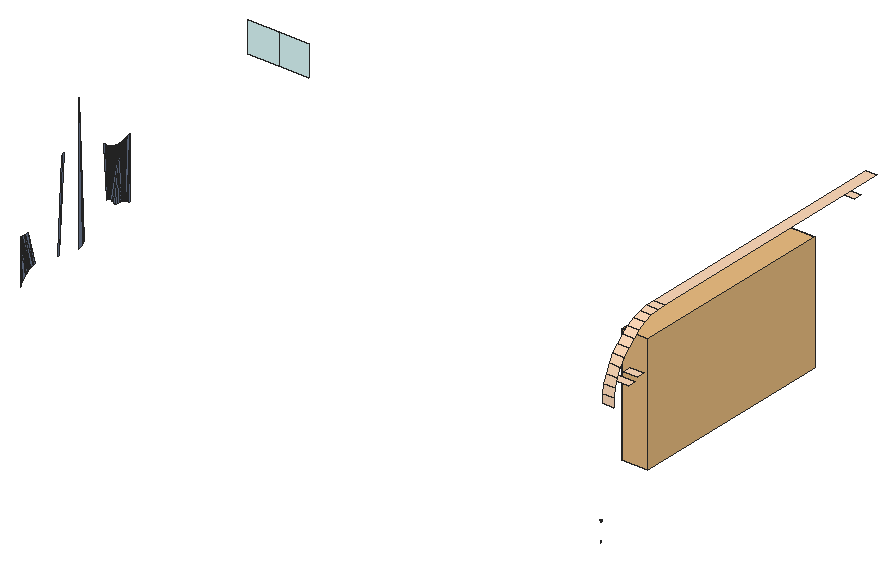
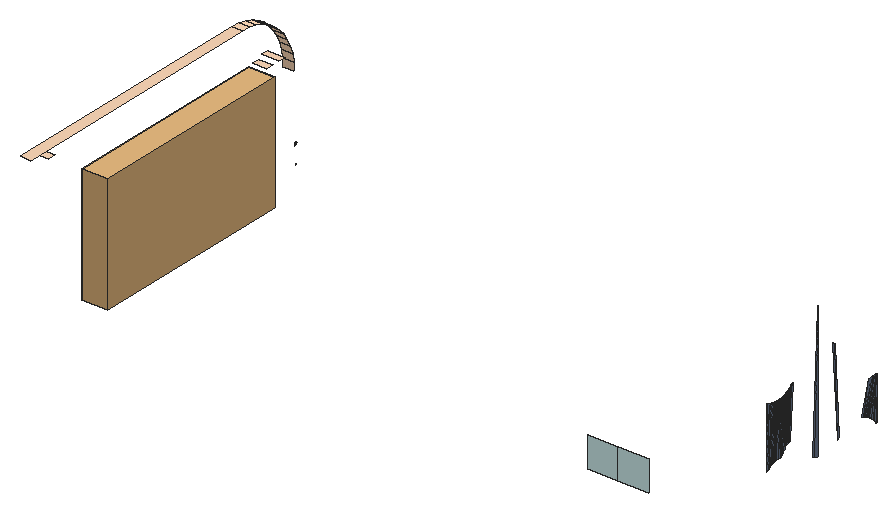
# SketchUp Ruby script. Lengths in inches.
U = 1.inch
M = Sketchup.active_model
def pt(a) = Geom::Point3d.new(a.map { |v| v * U })
def face(e, loops, mat)
  f = e.add_face(loops[0].map { |a| pt(a) })
  loops[1..].each { |l| e.add_face(l.map { |a| pt(a) }).erase! }
  f.material = f.back_material = mat if mat
  f
end
# faces: each face lists its corners as indices into pts; further lists are holes
def faces(e, pts, list, mat = nil) = list.each { |f| face(e, (f[0].is_a?(Array) ? f : [f]).map { |l| l.map { |i| pts[i] } }, mat) }
# xy, xz, yz: faces in a plane at the given z, y or x. An outline is a flat list of corners, or four numbers for a rectangle; further outlines are holes
def ring(l) = l.size == 4 ? [[l[0], l[1]], [l[2], l[1]], [l[2], l[3]], [l[0], l[3]]] : l.each_slice(2).to_a
def flat(e, list, mat, &to3) = list.each { |f| face(e, (f[0].is_a?(Array) ? f : [f]).map { |l| ring(l).map { |u, v| to3.(u, v) } }, mat) }
def xy(e, z, list, mat = nil) = flat(e, list, mat) { |x, y| [x, y, z] }
def xz(e, y, list, mat = nil) = flat(e, list, mat) { |x, z| [x, y, z] }
def yz(e, x, list, mat = nil) = flat(e, list, mat) { |y, z| [x, y, z] }
def lines(e, pts, list) = list.each { |a, b| e.add_line(pt(pts[a]), pt(pts[b])) }
# prism: a flat outline (further loops are holes) pulled along v
def prism(e, loops, v, mat = nil)
  f = face(e, loops, mat); d = Geom::Vector3d.new(v.map { |x| x * U })
  f.pushpull(f.normal.samedirection?(d) ? d.length : -d.length)
end
def box(e, o, s, mat = nil) = prism(e, [[o, [o[0] + s[0], o[1], o[2]], [o[0] + s[0], o[1] + s[1], o[2]], [o[0], o[1] + s[1], o[2]]]], [0, 0, s[2]], mat)
def at(x, y, z, deg = 0) = Geom::Transformation.translation(pt([x, y, z])) * Geom::Transformation.rotation(ORIGIN, Z_AXIS, deg.degrees)
def axes(o, x, y, z) = Geom::Transformation.new([*x, 0, *y, 0, *z, 0, *pt(o).to_a, 1])
def part(name) = M.definitions.add(name)
# library, detail: a bought-in or finely detailed component or shape, given as its bounding box
def library(name, o, s) = part(name).tap { |d| box(d.entities, o, s) }
def detail(e, o, s) = box(e.add_group.entities, o, s)
def put(e, d, t, mat = nil) = e.add_instance(d, t).tap { |i| i.material = mat if mat }
def group(e, t, mat = nil) = e.add_group.tap { |g| g.transformation = t; g.material = mat if mat }.entities
root = M.entities
M.materials.add("3D66_SU_1584934530605_002").color = [112, 126, 151]
M.materials.add("Material \#1").color = [140, 140, 140]
M.materials.add("[0027_PeachPuff]").color = [255, 218, 185]
M.materials.add("[0090_LightCyan]").color = [224, 255, 255]
c1 = library("Flat screen television",[0,1.41,1.14],[35.92,0.28,20.21])
xy(root,94.84,[[354.3125,217.7,361.25,220.7],[354.3125,223.77,359.875,226.77]],"[0027_PeachPuff]")
xy(root,110.27,[[354.3125,330.97,359.375,333.97]],"[0027_PeachPuff]")
xy(root,113.35,[[354.3125,238.49,358.5625,342.58]],"[0027_PeachPuff]")
xz(root,333.9375,[[118.5625,75.41,130.5625,87.41],[130.5625,75.41,142.5625,87.41]],"[0090_LightCyan]")
yz(root,123.07,[[216.34,46.75,216.58,47.05,216.82,47.36],[216.34,46.75,216.82,47.36,216.34,64.1875],[216.82,47.36,217.29,47.98,216.34,64.1875],[216.82,47.36,217.06,47.67,217.29,47.98],[244.87,47.51,246.34,48.07,244.87,100.53],
  [217.29,47.98,217.81,48.58,216.34,64.1875],[217.29,47.98,217.54,48.28,217.81,48.58],[246.34,48.07,247.03,48.37,244.87,100.53],[247.03,48.37,247.68,48.68,244.87,100.53],[217.81,48.58,218.42,49.17,216.34,64.1875],
  [217.81,48.58,218.1,48.875,218.42,49.17],[218.42,49.17,219.12,49.77,216.34,64.1875],[218.42,49.17,218.76,49.47,219.12,49.77],[235.3125,49.2,236.83,83.75,234.68,49.63],[235.3125,49.2,237.76,84.43,236.83,83.75],
  [219.12,49.77,219.86,50.33,216.34,64.1875],[219.12,49.77,219.49,50.06,219.86,50.33],[219.86,50.33,220.23,50.58,216.34,64.1875],[220.23,50.58,216.63,64.11,216.34,64.1875],[220.23,50.58,220.59,50.81,216.63,64.11],
  [220.59,50.81,216.92,64.05,216.63,64.11],[220.59,50.81,220.9375,51.01,216.92,64.05],[220.9375,51.01,217.23,63.99,216.92,64.05],[220.9375,51.01,217.84,63.92,217.23,63.99],[220.9375,51.01,218.15,63.9,217.84,63.92],
  [220.9375,51.01,221.3,51.18,218.15,63.9],[221.3,51.18,218.47,63.89,218.15,63.9],[221.3,51.18,221.65,51.34,218.47,63.89],[221.65,51.34,222.35,51.6,218.47,63.89],[221.65,51.34,222,51.48,222.35,51.6],
  [222.35,51.6,222.6875,51.7,218.47,63.89],[222.6875,51.7,220.09,64.05,218.47,63.89],[222.6875,51.7,223.3125,51.87,220.09,64.05],[222.6875,51.7,223.01,51.79,223.3125,51.87],[269.95,53.02,269.95,77.01,269.54,53.4],
  [269.54,53.4,269.95,77.01,269.33,53.58],[269.33,53.58,269.95,77.01,269.11,53.75],[269.11,53.75,269.95,77.01,268.89,53.9],[268.89,53.9,269.95,77.01,268.66,54.05],[268.19,54.33,269.95,77.01,268.79,76.57],
  [267.48,54.67,268.79,76.57,268.2,76.37],[267.23,54.76,268.2,76.37,267.6,76.18],[266.71,54.93,267.6,76.18,266.99,76.03],[266.43,55,266.68,75.97,266.13,55.07],[266.43,55,266.99,76.03,266.68,75.97],
  [266.13,55.07,266.37,75.91,266.05,55.09],[266.13,55.07,266.68,75.97,266.37,75.91],[266.05,55.09,266.37,75.91,265.97,55.1],[265.97,55.1,266.05,75.87,265.79,55.12],[265.97,55.1,266.37,75.91,266.05,75.87],
  [265.79,55.12,265.72,75.84,265.61,55.13],[265.79,55.12,266.05,75.87,265.72,75.84],[265.61,55.13,265.4,75.82,265.43,55.14],[265.61,55.13,265.72,75.84,265.4,75.82],[265.43,55.14,265.06,75.81,264.64,55.15],
  [265.43,55.14,265.4,75.82,265.06,75.81],[264.64,55.15,265.06,75.81,264.24,55.16],[264.24,55.16,265.06,75.81,264.05,55.18],[264.05,55.18,265.06,75.81,263.86,55.2],[263.86,55.2,265.06,75.81,263.76,55.22],
  [263.76,55.22,265.06,75.81,263.67,55.24],[263.67,55.24,265.06,75.81,263.58,55.26],[263.58,55.26,265.06,75.81,263.49,55.28],[263.49,55.28,265.06,75.81,263.41,55.31],[263.41,55.31,265.06,75.81,263.32,55.34],
  [263.32,55.34,265.06,75.81,263.24,55.37],[263.24,55.37,265.06,75.81,263.16,55.41],[263.16,55.41,265.06,75.81,263.09,55.45],[263.09,55.45,265.06,75.81,263.01,55.5],[263.01,55.5,265.06,75.81,262.94,55.55],
  [262.94,55.55,265.06,75.81,262.87,55.61],[262.87,55.61,265.06,75.81,262.8,55.66],[262.8,55.66,265.06,75.81,262.73,55.73],[262.73,55.73,265.06,75.81,262.6,55.86],[262.6,55.86,265.06,75.81,262.47,56],
  [262.47,56,265.06,75.81,262.35,56.15],[262.35,56.15,265.06,75.81,262.11,56.47],[262.11,56.47,265.06,75.81,261.65,57.11],[261.65,57.11,265.06,75.81,261.53,57.26],[261.53,57.26,265.06,75.81,261.41,57.4],
  [261.41,57.4,265.06,75.81,261.29,57.52],[261.29,57.52,265.06,75.81,261.23,57.58],[261.23,57.58,265.06,75.81,261.17,57.64],[261.17,57.64,265.06,75.81,260.66,58.06],[260.66,58.06,265.06,75.81,260.4,58.25],
  [260.4,58.25,265.06,75.81,260.14,58.42],[260.14,58.42,265.06,75.81,259.88,58.58],[259.88,58.58,265.06,75.81,259.76,58.65],[259.76,58.65,265.06,75.81,259.63,58.71],[259.63,58.71,264.58,75.82,259.5,58.77],
  [259.63,58.71,265.06,75.81,264.58,75.82],[259.5,58.77,264.58,75.82,259.375,58.8125],[259.375,58.8125,264.1,75.85,259.25,58.85],[259.375,58.8125,264.58,75.82,264.1,75.85],[259.25,58.85,263.63,75.9,259.1875,58.87],
  [259.25,58.85,264.1,75.85,263.63,75.9],[259.1875,58.87,263.63,75.9,259.125,58.89],[259.125,58.89,263.17,75.97,259.07,58.9],[259.125,58.89,263.63,75.9,263.17,75.97],[259.07,58.9,263.17,75.97,259,58.91],
  [259,58.91,262.72,76.05,258.94,58.92],[259,58.91,263.17,75.97,262.72,76.05],[258.625,58.92,257.83,78.65,257.55,78.95],[258.625,58.92,258.12,78.37,257.83,78.65],[258.625,58.92,258.43,78.1,258.12,78.37],
  [258.625,58.92,258.76,77.84,258.43,78.1],[258.625,58.92,258.6875,58.93,261.84,76.28],[258.625,58.92,259.1,77.59,258.76,77.84],[258.625,58.92,259.45,77.36,259.1,77.59],[258.625,58.92,259.82,77.14,259.45,77.36],
  [258.625,58.92,260.2,76.94,259.82,77.14],[258.625,58.92,260.59,76.75,260.2,76.94],[258.625,58.92,261,76.58,260.59,76.75],[258.625,58.92,261.41,76.42,261,76.58],[258.625,58.92,261.84,76.28,261.41,76.42],
  [258.88,58.92,262.27,76.16,258.8125,58.93],[258.88,58.92,258.94,58.92,262.72,76.05],[258.88,58.92,262.72,76.05,262.27,76.16],[258.6875,58.93,258.75,58.93,261.84,76.28],[258.75,58.93,258.8125,58.93,262.27,76.16],
  [258.75,58.93,262.27,76.16,261.84,76.28],[217.84,63.92,217.53,63.95,217.23,63.99]],"3D66_SU_1584934530605_002")
yz(root,362.5625,[[201.98,47.07,201.99,47.07,202.1,47.3],[201.99,47.07,202.04,47.14,202.1,47.3],[202.04,47.14,202.07,47.17,202.08,47.21],[202.04,47.14,202.08,47.21,202.1,47.3],[202.01,47.15,202.1,47.3,202.04,47.21],
  [202.04,47.21,202.1,47.3,202.0625,47.27],[202.08,47.21,202.09,47.25,202.1,47.3],[202.0625,47.27,202.1,47.3,202.07,47.34],[202.1,47.3,202.04,47.55,202.0625,47.41],[202.1,47.3,202.1,47.42,202.04,47.55],
  [202.1,47.3,202.0625,47.41,202.07,47.34],[202.1,47.3,202.11,47.34,202.1,47.42]],"Material \#1")
yz(root,362.57,[[202.58,54.24,202.58,54.4,202.5625,54.4],[202.58,54.24,202.59,54.24,202.58,54.4],[202.5625,54.4,202.54,54.54,202.53,54.54],[202.5625,54.4,202.58,54.4,202.54,54.54],[202.02,54.44,202.04,54.49,202.01,54.45],
  [202.01,54.45,202.04,54.49,202.03,54.49],[202.03,54.49,202.04,54.49,202.06,54.54],[202.03,54.49,202.06,54.54,202.04,54.54],[202.04,54.54,202.06,54.54,202.0625,54.6],[202.04,54.54,202.0625,54.6,202.05,54.6],
  [202.53,54.54,202.48,54.68,202.47,54.67],[202.53,54.54,202.54,54.54,202.48,54.68],[202.05,54.6,202.06,54.64,202.04,54.64],[202.05,54.6,202.0625,54.6,202.06,54.64],[202.04,54.64,202.04,54.6875,202.03,54.68],
  [202.04,54.64,202.06,54.64,202.04,54.6875],[202.47,54.67,202.4,54.8,202.39,54.79],[202.47,54.67,202.48,54.68,202.4,54.8],[202.03,54.68,202.02,54.73,202.01,54.73],[202.03,54.68,202.04,54.6875,202.02,54.73],
  [202.39,54.79,202.31,54.9,202.3,54.89],[202.39,54.79,202.4,54.8,202.31,54.9],[202.3,54.89,202.2,54.99,202.19,54.98],[202.3,54.89,202.31,54.9,202.2,54.99],[202.19,54.98,202.07,55.05,202.07,55.04],
  [202.19,54.98,202.2,54.99,202.07,55.05],[202.07,55.04,202.07,55.05,201.94,55.09]],"Material \#1")
yz(root,362.58,[[201.98,47.0625,202.01,47.15,202.04,47.21],[201.98,47.0625,202.04,47.21,202.1,47.3],[201.98,47.0625,202.1,47.3,201.98,47.07],[201.98,47.07,202.1,47.3,201.99,47.07],[201.99,47.07,202.04,47.14,201.99,47.08],
  [201.99,47.07,202.1,47.3,202.04,47.14],[201.99,47.08,202.04,47.14,202.02,47.11],[202.04,47.14,202.08,47.21,202.07,47.17],[202.04,47.14,202.1,47.3,202.08,47.21],[202.04,47.21,202.0625,47.27,202.1,47.3],
  [202.08,47.21,202.1,47.3,202.09,47.25],[202.0625,47.27,202.07,47.34,202.1,47.3],[202.1,47.3,202.04,47.47,202.04,47.55],[202.1,47.3,202.04,47.55,202.1,47.42],[202.1,47.3,202.0625,47.41,202.04,47.47],
  [202.1,47.3,202.07,47.34,202.0625,47.41],[202.1,47.3,202.1,47.42,202.11,47.34],[202.1,47.42,202.04,47.55,202.07,47.49]],"Material \#1")
yz(root,362.67,[[201.98,47.0625,202.1,47.3,202.04,47.21],[201.98,47.07,201.99,47.07,202.1,47.3],[201.99,47.07,202.04,47.14,202.1,47.3],[202.04,47.14,202.07,47.17,202.08,47.21],[202.04,47.14,202.08,47.21,202.1,47.3],
  [202.04,47.21,202.1,47.3,202.0625,47.27],[202.08,47.21,202.09,47.25,202.1,47.3],[202.0625,47.27,202.1,47.3,202.07,47.34],[202.1,47.3,202.04,47.47,202.0625,47.41],[202.1,47.3,202.04,47.55,202.04,47.47],
  [202.1,47.3,202.1,47.42,202.04,47.55],[202.1,47.3,202.0625,47.41,202.07,47.34],[202.1,47.3,202.11,47.34,202.1,47.42],[202.1,47.42,202.07,47.49,202.04,47.55],[202.04,47.47,202.04,47.55,202.01,47.52]],"Material \#1")
yz(root,362.6875,[[201.98,47.07,202.1,47.3,201.99,47.07],[201.99,47.07,202.1,47.3,202.04,47.14],[202.04,47.14,202.08,47.21,202.07,47.17],[202.04,47.14,202.1,47.3,202.08,47.21],[202.01,47.15,202.04,47.21,202.1,47.3],
  [202.04,47.21,202.0625,47.27,202.1,47.3],[202.08,47.21,202.1,47.3,202.09,47.25],[202.0625,47.27,202.07,47.34,202.1,47.3],[202.1,47.3,202.04,47.55,202.1,47.42],[202.1,47.3,202.0625,47.41,202.04,47.55],
  [202.1,47.3,202.07,47.34,202.0625,47.41],[202.1,47.3,202.1,47.42,202.11,47.34],[202.0625,47.41,202.04,47.47,202.04,47.55],[202.1,47.42,202.04,47.55,202.07,47.49],[202.04,47.47,202.01,47.52,202.04,47.55]],"Material \#1")
yz(root,362.69,[[202.58,54.24,202.5625,54.4,202.58,54.4],[202.58,54.24,202.58,54.4,202.59,54.24],[202.5625,54.4,202.53,54.54,202.54,54.54],[202.5625,54.4,202.54,54.54,202.58,54.4],[202.02,54.44,202.01,54.45,202.04,54.49],
  [202.01,54.45,202.03,54.49,202.04,54.49],[202.03,54.49,202.04,54.54,202.06,54.54],[202.03,54.49,202.06,54.54,202.04,54.49],[202.04,54.54,202.05,54.6,202.0625,54.6],[202.04,54.54,202.0625,54.6,202.06,54.54],
  [202.53,54.54,202.47,54.67,202.48,54.68],[202.53,54.54,202.48,54.68,202.54,54.54],[202.05,54.6,202.04,54.64,202.06,54.64],[202.05,54.6,202.06,54.64,202.0625,54.6],[202.04,54.64,202.03,54.68,202.04,54.6875],
  [202.04,54.64,202.04,54.6875,202.06,54.64],[202.47,54.67,202.39,54.79,202.4,54.8],[202.47,54.67,202.4,54.8,202.48,54.68],[202.03,54.68,202.01,54.73,202.02,54.73],[202.03,54.68,202.02,54.73,202.04,54.6875],
  [202.39,54.79,202.3,54.89,202.31,54.9],[202.39,54.79,202.31,54.9,202.4,54.8],[202.3,54.89,202.19,54.98,202.2,54.99],[202.3,54.89,202.2,54.99,202.31,54.9],[202.19,54.98,202.07,55.04,202.07,55.05],
  [202.19,54.98,202.07,55.05,202.2,54.99],[202.07,55.04,201.94,55.09,202.07,55.05]],"Material \#1")
p = [[354.3125,213.59,91.51],[354.3125,213.375,88.23],[358.5625,213.375,88.23],[358.5625,213.59,91.51],[354.3125,214.23,94.73],[358.5625,214.23,94.73],
  [354.3125,215.29,97.85],[358.5625,215.29,97.85],[354.3125,216.74,100.79],[358.5625,216.74,100.79],[354.3125,218.57,103.52],[358.5625,218.57,103.52],
  [354.3125,220.73,106],[358.5625,220.73,106],[354.3125,223.2,108.16],[358.5625,223.2,108.16],[354.3125,225.93,109.99],[358.5625,225.93,109.99],
  [354.3125,228.88,111.44],[358.5625,228.88,111.44],[354.3125,231.99,112.5],[358.5625,231.99,112.5],[354.3125,235.22,113.14],[358.5625,235.22,113.14],
  [354.3125,238.49,113.35],[358.5625,238.49,113.35]]
faces(root,p,[[0,1,2,3],[4,0,3,5],[6,4,5,7],[8,6,7,9],[10,8,9,11],[12,10,11,13],[14,12,13,15],[16,14,15,17],
  [18,16,17,19],[20,18,19,21],[22,20,21,23],[24,22,23,25]],"[0027_PeachPuff]")
put(root,c1,axes([291.74,318.81,51.47],[0,-2.28327,0],[36.53232,0,0],[0,0,2.28327]))
